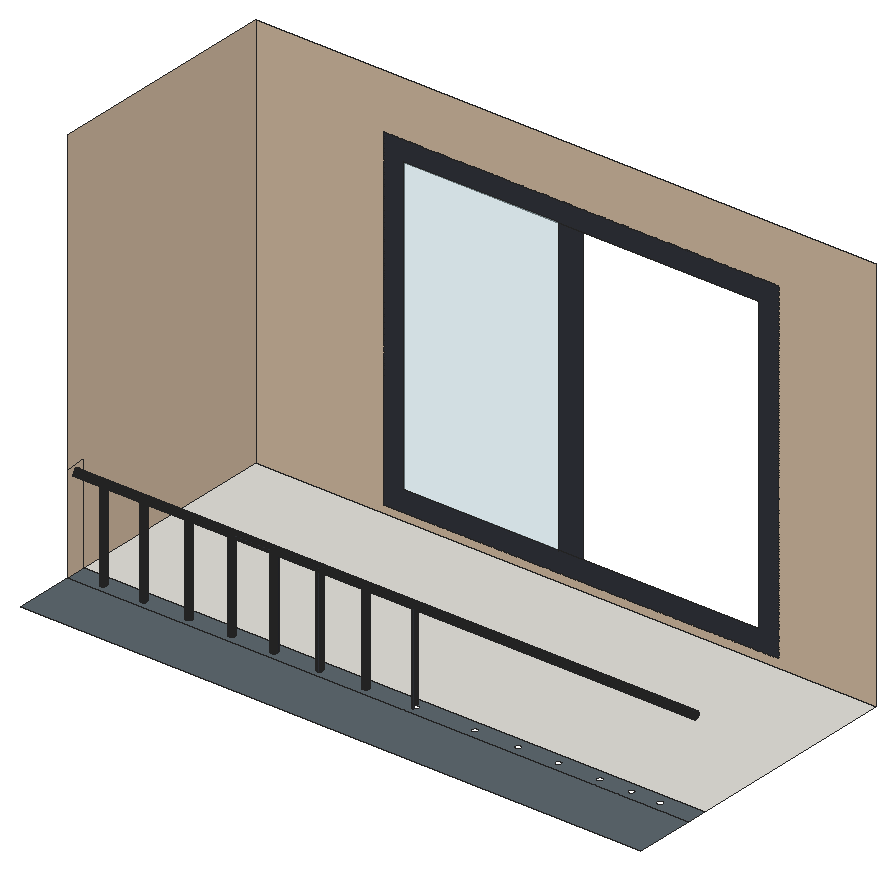
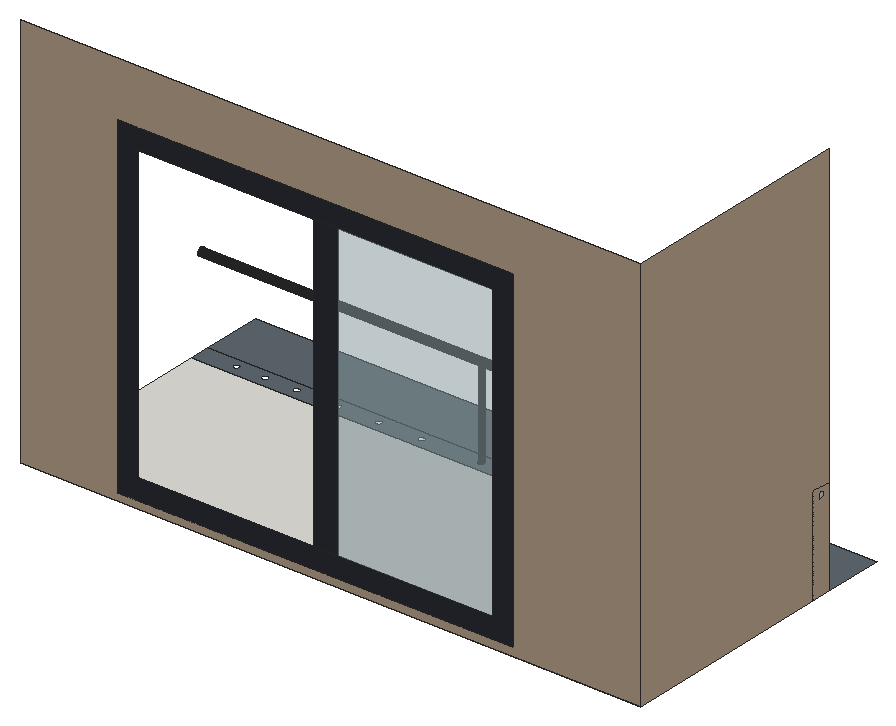
# SketchUp Ruby script. Lengths in inches.
U = 1.inch
M = Sketchup.active_model
def pt(a) = Geom::Point3d.new(a.map { |v| v * U })
def face(e, loops, mat)
  f = e.add_face(loops[0].map { |a| pt(a) })
  loops[1..].each { |l| e.add_face(l.map { |a| pt(a) }).erase! }
  f.material = f.back_material = mat if mat
  f
end
# faces: each face lists its corners as indices into pts; further lists are holes
def faces(e, pts, list, mat = nil) = list.each { |f| face(e, (f[0].is_a?(Array) ? f : [f]).map { |l| l.map { |i| pts[i] } }, mat) }
# xy, xz, yz: faces in a plane at the given z, y or x. An outline is a flat list of corners, or four numbers for a rectangle; further outlines are holes
def ring(l) = l.size == 4 ? [[l[0], l[1]], [l[2], l[1]], [l[2], l[3]], [l[0], l[3]]] : l.each_slice(2).to_a
def flat(e, list, mat, &to3) = list.each { |f| face(e, (f[0].is_a?(Array) ? f : [f]).map { |l| ring(l).map { |u, v| to3.(u, v) } }, mat) }
def xy(e, z, list, mat = nil) = flat(e, list, mat) { |x, y| [x, y, z] }
def xz(e, y, list, mat = nil) = flat(e, list, mat) { |x, z| [x, y, z] }
def yz(e, x, list, mat = nil) = flat(e, list, mat) { |y, z| [x, y, z] }
def lines(e, pts, list) = list.each { |a, b| e.add_line(pt(pts[a]), pt(pts[b])) }
# prism: a flat outline (further loops are holes) pulled along v
def prism(e, loops, v, mat = nil)
  f = face(e, loops, mat); d = Geom::Vector3d.new(v.map { |x| x * U })
  f.pushpull(f.normal.samedirection?(d) ? d.length : -d.length)
end
def box(e, o, s, mat = nil) = prism(e, [[o, [o[0] + s[0], o[1], o[2]], [o[0] + s[0], o[1] + s[1], o[2]], [o[0], o[1] + s[1], o[2]]]], [0, 0, s[2]], mat)
def at(x, y, z, deg = 0) = Geom::Transformation.translation(pt([x, y, z])) * Geom::Transformation.rotation(ORIGIN, Z_AXIS, deg.degrees)
def axes(o, x, y, z) = Geom::Transformation.new([*x, 0, *y, 0, *z, 0, *pt(o).to_a, 1])
def part(name) = M.definitions.add(name)
# library, detail: a bought-in or finely detailed component or shape, given as its bounding box
def library(name, o, s) = part(name).tap { |d| box(d.entities, o, s) }
def detail(e, o, s) = box(e.add_group.entities, o, s)
def put(e, d, t, mat = nil) = e.add_instance(d, t).tap { |i| i.material = mat if mat }
def group(e, t, mat = nil) = e.add_group.tap { |g| g.transformation = t; g.material = mat if mat }.entities
root = M.entities
M.materials.add("[Formica Laminate Dark]").color = [50, 53, 60]
M.materials.add("[Formica Laminate Light]").color = [213, 189, 164]
M.materials.add("[Formica Speckled Grey]").color = [94, 105, 111]
M.materials.add("[Marble Carrara Gold Floor Tile]").color = [225, 223, 217]
M.materials.add("[Translucent Glass Safety]").color = [204, 235, 244]
M.materials["[Translucent Glass Safety]"].alpha = 0.5
xy(root,133.5625,[[17.2,124.59,16.95,124.62,16.73,124.71,16.53,124.86,16.38,125.06,16.29,125.28,16.26,125.52,16.29,125.77,16.38,125.99,16.53,126.1875,16.73,126.34,16.95,126.43,17.2,126.46,17.4375,126.43,17.67,126.34,17.86,126.1875,18.01,125.99,18.1,125.77,18.13,125.52,18.1,125.28,18.01,125.06,17.86,124.86,17.67,124.71,17.4375,124.62],[29.01,124.59,28.77,124.62,28.54,124.71,28.35,124.86,28.2,125.06,28.1,125.28,28.07,125.52,28.1,125.77,28.2,125.99,28.35,126.1875,28.54,126.34,28.77,126.43,29.01,126.46,29.25,126.43,29.48,126.34,29.67,126.1875,29.82,125.99,29.91,125.77,29.95,125.52,29.91,125.28,29.82,125.06,29.67,124.86,29.48,124.71,29.25,124.62],[42.13,124.59,41.89,124.62,41.67,124.71,41.47,124.86,41.32,125.06,41.23,125.28,41.2,125.52,41.23,125.77,41.32,125.99,41.47,126.1875,41.67,126.34,41.89,126.43,42.13,126.46,42.375,126.43,42.6,126.34,42.8,126.1875,42.95,125.99,43.04,125.77,43.07,125.52,43.04,125.28,42.95,125.06,42.8,124.86,42.6,124.71,42.375,124.62],[54.63,124.59,54.39,124.62,54.17,124.71,53.97,124.86,53.82,125.06,53.73,125.28,53.7,125.52,53.73,125.77,53.82,125.99,53.97,126.1875,54.17,126.34,54.39,126.43,54.63,126.46,54.875,126.43,55.1,126.34,55.3,126.1875,55.45,125.99,55.54,125.77,55.57,125.52,55.54,125.28,55.45,125.06,55.3,124.86,55.1,124.71,54.875,124.62],[66.88,124.59,66.64,124.62,66.42,124.71,66.22,124.86,66.07,125.06,65.98,125.28,65.95,125.52,65.98,125.77,66.07,125.99,66.22,126.1875,66.42,126.34,66.64,126.43,66.88,126.46,67.125,126.43,67.35,126.34,67.55,126.1875,67.7,125.99,67.79,125.77,67.82,125.52,67.79,125.28,67.7,125.06,67.55,124.86,67.35,124.71,67.125,124.62],
  [80.2,124.59,79.95,124.62,79.73,124.71,79.53,124.86,79.38,125.06,79.29,125.28,79.26,125.52,79.29,125.77,79.38,125.99,79.53,126.1875,79.73,126.34,79.95,126.43,80.2,126.46,80.4375,126.43,80.67,126.34,80.86,126.1875,81.01,125.99,81.1,125.77,81.13,125.52,81.1,125.28,81.01,125.06,80.86,124.86,80.67,124.71,80.4375,124.62],[93.63,124.59,93.39,124.62,93.17,124.71,92.97,124.86,92.82,125.06,92.73,125.28,92.7,125.52,92.73,125.77,92.82,125.99,92.97,126.1875,93.17,126.34,93.39,126.43,93.63,126.46,93.875,126.43,94.1,126.34,94.3,126.1875,94.45,125.99,94.54,125.77,94.57,125.52,94.54,125.28,94.45,125.06,94.3,124.86,94.1,124.71,93.875,124.62]])
xy(root,133.5625,[[9,105.54,189.57,122.79],[[9,122.79,189.57,128.69],[179.2,124.59,178.95,124.62,178.73,124.71,178.53,124.86,178.38,125.06,178.29,125.28,178.26,125.52,178.29,125.77,178.38,125.99,178.53,126.1875,178.73,126.34,178.95,126.43,179.2,126.46,179.4375,126.43,179.67,126.34,179.86,126.1875,180.01,125.99,180.1,125.77,180.13,125.52,180.1,125.28,180.01,125.06,179.86,124.86,179.67,124.71,179.4375,124.62],[29.01,124.59,28.77,124.62,28.54,124.71,28.35,124.86,28.2,125.06,28.1,125.28,28.07,125.52,28.1,125.77,28.2,125.99,28.35,126.1875,28.54,126.34,28.77,126.43,29.01,126.46,29.25,126.43,29.48,126.34,29.67,126.1875,29.82,125.99,29.91,125.77,29.95,125.52,29.91,125.28,29.82,125.06,29.67,124.86,29.48,124.71,29.25,124.62],[161.7,124.59,161.45,124.62,161.23,124.71,161.03,124.86,160.88,125.06,160.79,125.28,160.76,125.52,160.79,125.77,160.88,125.99,161.03,126.1875,161.23,126.34,161.45,126.43,161.7,126.46,161.9375,126.43,162.17,126.34,162.36,126.1875,162.51,125.99,162.6,125.77,162.63,125.52,162.6,125.28,162.51,125.06,162.36,124.86,162.17,124.71,161.9375,124.62],[42.13,124.59,41.89,124.62,41.67,124.71,41.47,124.86,41.32,125.06,41.23,125.28,41.2,125.52,41.23,125.77,41.32,125.99,41.47,126.1875,41.67,126.34,41.89,126.43,42.13,126.46,42.375,126.43,42.6,126.34,42.8,126.1875,42.95,125.99,43.04,125.77,43.07,125.52,43.04,125.28,42.95,125.06,42.8,124.86,42.6,124.71,42.375,124.62],[149.57,124.59,149.33,124.62,149.1,124.71,148.91,124.86,148.76,125.06,148.67,125.28,148.63,125.52,148.67,125.77,148.76,125.99,148.91,126.1875,149.1,126.34,149.33,126.43,149.57,126.46,149.8125,126.43,150.04,126.34,150.23,126.1875,150.38,125.99,150.48,125.77,150.51,125.52,150.48,125.28,150.38,125.06,150.23,124.86,150.04,124.71,149.8125,124.62],[54.63,124.59,54.39,124.62,54.17,124.71,53.97,124.86,53.82,125.06,53.73,125.28,53.7,125.52,53.73,125.77,53.82,125.99,53.97,126.1875,54.17,126.34,54.39,126.43,54.63,126.46,54.875,126.43,55.1,126.34,55.3,126.1875,55.45,125.99,55.54,125.77,55.57,125.52,55.54,125.28,55.45,125.06,55.3,124.86,55.1,124.71,54.875,124.62],[137.76,124.59,137.52,124.62,137.29,124.71,137.1,124.86,136.95,125.06,136.85,125.28,136.82,125.52,136.85,125.77,136.95,125.99,137.1,126.1875,137.29,126.34,137.52,126.43,137.76,126.46,138,126.43,138.23,126.34,138.42,126.1875,138.57,125.99,138.66,125.77,138.7,125.52,138.66,125.28,138.57,125.06,138.42,124.86,138.23,124.71,138,124.62],[66.88,124.59,66.64,124.62,66.42,124.71,66.22,124.86,66.07,125.06,65.98,125.28,65.95,125.52,65.98,125.77,66.07,125.99,66.22,126.1875,66.42,126.34,66.64,126.43,66.88,126.46,67.125,126.43,67.35,126.34,67.55,126.1875,67.7,125.99,67.79,125.77,67.82,125.52,67.79,125.28,67.7,125.06,67.55,124.86,67.35,124.71,67.125,124.62],[125.32,124.59,125.08,124.62,124.85,124.71,124.66,124.86,124.51,125.06,124.42,125.28,124.38,125.52,124.42,125.77,124.51,125.99,124.66,126.1875,124.85,126.34,125.08,126.43,125.32,126.46,125.5625,126.43,125.79,126.34,125.98,126.1875,126.13,125.99,126.23,125.77,126.26,125.52,126.23,125.28,126.13,125.06,125.98,124.86,125.79,124.71,125.5625,124.62],[80.2,124.59,79.95,124.62,79.73,124.71,79.53,124.86,79.38,125.06,79.29,125.28,79.26,125.52,79.29,125.77,79.38,125.99,79.53,126.1875,79.73,126.34,79.95,126.43,80.2,126.46,80.4375,126.43,80.67,126.34,80.86,126.1875,81.01,125.99,81.1,125.77,81.13,125.52,81.1,125.28,81.01,125.06,80.86,124.86,80.67,124.71,80.4375,124.62],[108.2,124.59,107.95,124.62,107.73,124.71,107.53,124.86,107.38,125.06,107.29,125.28,107.26,125.52,107.29,125.77,107.38,125.99,107.53,126.1875,107.73,126.34,107.95,126.43,108.2,126.46,108.4375,126.43,108.67,126.34,108.86,126.1875,109.01,125.99,109.1,125.77,109.13,125.52,109.1,125.28,109.01,125.06,108.86,124.86,108.67,124.71,108.4375,124.62],[93.63,124.59,93.39,124.62,93.17,124.71,92.97,124.86,92.82,125.06,92.73,125.28,92.7,125.52,92.73,125.77,92.82,125.99,92.97,126.1875,93.17,126.34,93.39,126.43,93.63,126.46,93.875,126.43,94.1,126.34,94.3,126.1875,94.45,125.99,94.54,125.77,94.57,125.52,94.54,125.28,94.45,125.06,94.3,124.86,94.1,124.71,93.875,124.62],[170.82,124.59,170.58,124.62,170.35,124.71,170.16,124.86,170.01,125.06,169.92,125.28,169.88,125.52,169.92,125.77,170.01,125.99,170.16,126.1875,170.35,126.34,170.58,126.43,170.82,126.46,171.0625,126.43,171.29,126.34,171.48,126.1875,171.63,125.99,171.73,125.77,171.76,125.52,171.73,125.28,171.63,125.06,171.48,124.86,171.29,124.71,171.0625,124.62],[17.2,124.59,16.95,124.62,16.73,124.71,16.53,124.86,16.38,125.06,16.29,125.28,16.26,125.52,16.29,125.77,16.38,125.99,16.53,126.1875,16.73,126.34,16.95,126.43,17.2,126.46,17.4375,126.43,17.67,126.34,17.86,126.1875,18.01,125.99,18.1,125.77,18.13,125.52,18.1,125.28,18.01,125.06,17.86,124.86,17.67,124.71,17.4375,124.62]]],"[Formica Speckled Grey]")
xy(root,133.5625,[[9,128.69,189.57,191.15]],"[Marble Carrara Gold Floor Tile]")
xy(root,159.8125,[[29.01,124.59,29.25,124.62,29.48,124.71,29.67,124.86,29.82,125.06,29.91,125.28,29.95,125.52,29.91,125.77,29.82,125.99,29.67,126.1875,29.48,126.34,29.25,126.43,29.01,126.46,28.77,126.43,28.54,126.34,28.35,126.1875,28.2,125.99,28.1,125.77,28.07,125.52,28.1,125.28,28.2,125.06,28.35,124.86,28.54,124.71,28.77,124.62]])
xy(root,159.9375,[[93.63,124.59,93.875,124.62,94.1,124.71,94.3,124.86,94.45,125.06,94.54,125.28,94.57,125.52,94.54,125.77,94.45,125.99,94.3,126.1875,94.1,126.34,93.875,126.43,93.63,126.46,93.39,126.43,93.17,126.34,92.97,126.1875,92.82,125.99,92.73,125.77,92.7,125.52,92.73,125.28,92.82,125.06,92.97,124.86,93.17,124.71,93.39,124.62]])
xy(root,160.19,[[54.63,124.59,54.78,124.61,54.49,124.61],[66.88,124.59,67.03,124.61,66.74,124.61],[54.49,124.61,54.78,124.61,54.875,124.62,55.1,124.71,55.3,124.86,55.45,125.06,55.54,125.28,55.57,125.52,55.54,125.77,55.45,125.99,55.3,126.1875,55.1,126.34,54.875,126.43,54.63,126.46,54.39,126.43,54.17,126.34,53.97,126.1875,53.82,125.99,53.73,125.77,53.7,125.52,53.73,125.28,53.82,125.06,53.97,124.86,54.17,124.71,54.39,124.62],[66.74,124.61,67.03,124.61,67.125,124.62,67.35,124.71,67.55,124.86,67.7,125.06,67.79,125.28,67.82,125.52,67.79,125.77,67.7,125.99,67.55,126.1875,67.35,126.34,67.125,126.43,66.88,126.46,66.64,126.43,66.42,126.34,66.22,126.1875,66.07,125.99,65.98,125.77,65.95,125.52,65.98,125.28,66.07,125.06,66.22,124.86,66.42,124.71,66.64,124.62]])
xy(root,160.25,[[42.13,124.59,42.375,124.62,42.6,124.71,42.8,124.86,42.95,125.06,43.04,125.28,43.07,125.52,43.04,125.77,42.95,125.99,42.8,126.1875,42.6,126.34,42.375,126.43,42.13,126.46,41.89,126.43,41.67,126.34,41.47,126.1875,41.32,125.99,41.23,125.77,41.2,125.52,41.23,125.28,41.32,125.06,41.47,124.86,41.67,124.71,41.89,124.62]])
xy(root,160.4375,[[17.2,124.59,17.4375,124.62,17.67,124.71,17.86,124.86,18.01,125.06,18.1,125.28,18.13,125.52,18.1,125.77,18.01,125.99,17.86,126.1875,17.67,126.34,17.4375,126.43,17.2,126.46,16.95,126.43,16.73,126.34,16.53,126.1875,16.38,125.99,16.29,125.77,16.26,125.52,16.29,125.28,16.38,125.06,16.53,124.86,16.73,124.71,16.95,124.62]])
xy(root,160.625,[[80.2,124.59,80.4375,124.62,80.67,124.71,80.86,124.86,81.01,125.06,81.1,125.28,81.13,125.52,81.1,125.77,81.01,125.99,80.86,126.1875,80.67,126.34,80.4375,126.43,80.2,126.46,79.95,126.43,79.73,126.34,79.53,126.1875,79.38,125.99,79.29,125.77,79.26,125.52,79.29,125.28,79.38,125.06,79.53,124.86,79.73,124.71,79.95,124.62]])
xz(root,191.15,[[[46.38,135.91,161.13,233.1],[52.18,141.71,155.34,227.3]],[97.09,141.71,104.16,227.3]],"[Formica Laminate Dark]")
xz(root,191.15,[[[9,133.5625,189.57,249],[46.38,135.91,161.13,233.1]]],"[Formica Laminate Light]")
xz(root,191.15,[[52.18,141.71,97.09,227.3]],"[Translucent Glass Safety]")
yz(root,9,[[125.67,159.02,125.41,159.03,125.16,159.11,124.94,159.25,124.77,159.45,124.65,159.68,124.59,159.93,124.61,160.19,124.6875,160.44,124.83,160.66,125.02,160.84,125.26,160.96,125.51,161.01,125.77,161,126.02,160.92,126.24,160.77,126.41,160.58,126.53,160.35,126.59,160.09,126.57,159.83,126.49,159.58,126.35,159.36,126.16,159.1875,125.92,159.07]])
yz(root,9,[[128.69,133.5625,191.15,133.5625,191.15,249,122.79,249,122.79,161.92,128.69,162.3125],[[122.79,133.5625,128.69,133.5625,128.69,162.3125,122.79,161.92],[125.67,159.02,125.41,159.03,125.16,159.11,124.94,159.25,124.77,159.45,124.65,159.68,124.59,159.93,124.61,160.19,124.6875,160.44,124.83,160.66,125.02,160.84,125.26,160.96,125.51,161.01,125.77,161,126.02,160.92,126.24,160.77,126.41,160.58,126.53,160.35,126.59,160.09,126.57,159.83,126.49,159.58,126.35,159.36,126.16,159.1875,125.92,159.07]]],"[Formica Laminate Light]")
p = [[16.73,124.71,133.5625],[16.95,124.62,133.5625],[16.95,124.62,160.4375],[16.73,124.71,160.4375],[17.2,124.59,133.5625],[17.2,124.59,160.4375],
  [17.4375,124.62,133.5625],[17.4375,124.62,160.4375],[17.67,124.71,133.5625],[17.67,124.71,160.4375],[28.54,124.71,133.5625],[28.77,124.62,133.5625],
  [28.77,124.62,159.8125],[28.54,124.71,159.8125],[29.01,124.59,133.5625],[29.01,124.59,159.8125],[29.25,124.62,133.5625],[29.25,124.62,159.8125],
  [29.48,124.71,133.5625],[29.48,124.71,159.8125],[41.67,124.71,133.5625],[41.89,124.62,133.5625],[41.89,124.62,160.25],[41.67,124.71,160.25],
  [42.13,124.59,133.5625],[42.13,124.59,160.25],[42.375,124.62,133.5625],[42.375,124.62,160.25],[42.6,124.71,133.5625],[42.6,124.71,160.25],
  [54.17,124.71,133.5625],[54.39,124.62,133.5625],[54.39,124.62,160.19],[54.17,124.71,160.19],[54.63,124.59,133.5625],[54.63,124.59,160.19],
  [54.49,124.61,160.19],[54.875,124.62,133.5625],[54.875,124.62,160.19],[54.78,124.61,160.19],[55.1,124.71,133.5625],[55.1,124.71,160.19],
  [66.42,124.71,133.5625],[66.64,124.62,133.5625],[66.64,124.62,160.19],[66.42,124.71,160.19],[66.88,124.59,133.5625],[66.88,124.59,160.19],
  [66.74,124.61,160.19],[67.125,124.62,133.5625],[67.125,124.62,160.19],[67.03,124.61,160.19],[67.35,124.71,133.5625],[67.35,124.71,160.19],
  [79.73,124.71,133.5625],[79.95,124.62,133.5625],[79.95,124.62,160.625],[79.73,124.71,160.625],[80.2,124.59,133.5625],[80.2,124.59,160.625],
  [80.4375,124.62,133.5625],[80.4375,124.62,160.625],[80.67,124.71,133.5625],[80.67,124.71,160.625],[93.17,124.71,133.5625],[93.39,124.62,133.5625],
  [93.39,124.62,159.9375],[93.17,124.71,159.9375],[93.63,124.59,133.5625],[93.63,124.59,159.9375],[93.875,124.62,133.5625],[93.875,124.62,159.9375],
  [94.1,124.71,133.5625],[94.1,124.71,159.9375],[107.73,124.71,133.5625],[107.95,124.62,133.5625],[107.95,124.62,160.125],[107.73,124.71,160.125],
  [108.2,124.59,133.5625],[108.2,124.59,160.125],[16.53,124.86,133.5625],[16.53,124.86,160.4375],[17.86,124.86,133.5625],[17.86,124.86,160.4375],
  [28.35,124.86,133.5625],[28.35,124.86,159.8125],[29.67,124.86,133.5625],[29.67,124.86,159.8125],[41.47,124.86,133.5625],[41.47,124.86,160.25],
  [42.8,124.86,133.5625],[42.8,124.86,160.25],[53.97,124.86,133.5625],[53.97,124.86,160.19],[55.3,124.86,133.5625],[55.3,124.86,160.19],
  [66.22,124.86,133.5625],[66.22,124.86,160.19],[67.55,124.86,133.5625],[67.55,124.86,160.19],[79.53,124.86,133.5625],[79.53,124.86,160.625],
  [80.86,124.86,133.5625],[80.86,124.86,160.625],[92.97,124.86,133.5625],[92.97,124.86,159.9375],[94.3,124.86,133.5625],[94.3,124.86,159.9375],
  [107.53,124.86,133.5625],[107.53,124.86,160.125],[16.38,125.06,133.5625],[16.38,125.06,160.4375],[18.01,125.06,133.5625],[18.01,125.06,160.4375],
  [28.2,125.06,133.5625],[28.2,125.06,159.8125],[29.82,125.06,133.5625],[29.82,125.06,159.8125],[41.32,125.06,133.5625],[41.32,125.06,160.25],
  [42.95,125.06,133.5625],[42.95,125.06,160.25],[53.82,125.06,133.5625],[53.82,125.06,160.19],[55.45,125.06,133.5625],[55.45,125.06,160.19],
  [66.07,125.06,133.5625],[66.07,125.06,160.19],[67.7,125.06,133.5625],[67.7,125.06,160.19],[79.38,125.06,133.5625],[79.38,125.06,160.625],
  [81.01,125.06,133.5625],[81.01,125.06,160.625],[92.82,125.06,133.5625],[92.82,125.06,159.9375],[94.45,125.06,133.5625],[94.45,125.06,159.9375],
  [107.38,125.06,133.5625],[107.38,125.06,160.125],[16.29,125.28,133.5625],[16.29,125.28,160.4375],[18.1,125.28,133.5625],[18.1,125.28,160.4375],
  [28.1,125.28,133.5625],[28.1,125.28,159.8125],[29.91,125.28,133.5625],[29.91,125.28,159.8125],[41.23,125.28,133.5625],[41.23,125.28,160.25],
  [43.04,125.28,133.5625],[43.04,125.28,160.25],[53.73,125.28,133.5625],[53.73,125.28,160.19],[55.54,125.28,133.5625],[55.54,125.28,160.19],
  [65.98,125.28,133.5625],[65.98,125.28,160.19],[67.79,125.28,133.5625],[67.79,125.28,160.19],[79.29,125.28,133.5625],[79.29,125.28,160.625],
  [81.1,125.28,133.5625],[81.1,125.28,160.625],[92.73,125.28,133.5625],[92.73,125.28,159.9375],[94.54,125.28,133.5625],[94.54,125.28,159.9375],
  [107.29,125.28,133.5625],[107.29,125.28,160.125],[16.26,125.52,133.5625],[16.26,125.52,160.4375],[18.13,125.52,133.5625],[18.13,125.52,160.4375],
  [28.07,125.52,133.5625],[28.07,125.52,159.8125],[29.95,125.52,133.5625],[29.95,125.52,159.8125],[41.2,125.52,133.5625],[41.2,125.52,160.25],
  [43.07,125.52,133.5625],[43.07,125.52,160.25],[53.7,125.52,133.5625],[53.7,125.52,160.19],[55.57,125.52,133.5625],[55.57,125.52,160.19],
  [65.95,125.52,133.5625],[65.95,125.52,160.19],[67.82,125.52,133.5625],[67.82,125.52,160.19],[79.26,125.52,133.5625],[79.26,125.52,160.625],
  [81.13,125.52,133.5625],[81.13,125.52,160.625],[92.7,125.52,133.5625],[92.7,125.52,159.9375],[94.57,125.52,133.5625],[94.57,125.52,159.9375],
  [107.26,125.52,133.5625],[107.26,125.52,160.125],[16.29,125.77,133.5625],[16.29,125.77,160.4375],[18.1,125.77,133.5625],[18.1,125.77,160.4375],
  [28.1,125.77,133.5625],[28.1,125.77,159.8125],[29.91,125.77,133.5625],[29.91,125.77,159.8125],[41.23,125.77,133.5625],[41.23,125.77,160.25],
  [43.04,125.77,133.5625],[43.04,125.77,160.25],[53.73,125.77,133.5625],[53.73,125.77,160.19],[55.54,125.77,133.5625],[55.54,125.77,160.19],
  [65.98,125.77,133.5625],[65.98,125.77,160.19],[67.79,125.77,133.5625],[67.79,125.77,160.19],[79.29,125.77,133.5625],[79.29,125.77,160.625],
  [81.1,125.77,133.5625],[81.1,125.77,160.625],[92.73,125.77,133.5625],[92.73,125.77,159.9375],[94.54,125.77,133.5625],[94.54,125.77,159.9375],
  [107.29,125.77,133.5625],[107.29,125.77,160.125],[16.38,125.99,133.5625],[16.38,125.99,160.4375],[18.01,125.99,133.5625],[18.01,125.99,160.4375],
  [28.2,125.99,133.5625],[28.2,125.99,159.8125],[29.82,125.99,133.5625],[29.82,125.99,159.8125],[41.32,125.99,133.5625],[41.32,125.99,160.25],
  [42.95,125.99,133.5625],[42.95,125.99,160.25],[53.82,125.99,133.5625],[53.82,125.99,160.19],[55.45,125.99,133.5625],[55.45,125.99,160.19],
  [66.07,125.99,133.5625],[66.07,125.99,160.19],[67.7,125.99,133.5625],[67.7,125.99,160.19],[79.38,125.99,133.5625],[79.38,125.99,160.625],
  [81.01,125.99,133.5625],[81.01,125.99,160.625],[92.82,125.99,133.5625],[92.82,125.99,159.9375],[94.45,125.99,133.5625],[94.45,125.99,159.9375],
  [107.38,125.99,133.5625],[107.38,125.99,160.125],[16.53,126.1875,133.5625],[16.53,126.1875,160.4375],[17.86,126.1875,133.5625],[17.86,126.1875,160.4375],
  [28.35,126.1875,133.5625],[28.35,126.1875,159.8125],[29.67,126.1875,133.5625],[29.67,126.1875,159.8125],[41.47,126.1875,133.5625],[41.47,126.1875,160.25],
  [42.8,126.1875,133.5625],[42.8,126.1875,160.25],[53.97,126.1875,133.5625],[53.97,126.1875,160.19],[55.3,126.1875,133.5625],[55.3,126.1875,160.19],
  [66.22,126.1875,133.5625],[66.22,126.1875,160.19],[67.55,126.1875,133.5625],[67.55,126.1875,160.19],[79.53,126.1875,133.5625],[79.53,126.1875,160.625],
  [80.86,126.1875,133.5625],[80.86,126.1875,160.625],[92.97,126.1875,133.5625],[92.97,126.1875,159.9375],[94.3,126.1875,133.5625],[94.3,126.1875,159.9375],
  [107.53,126.1875,133.5625],[107.53,126.1875,160.125],[16.73,126.34,133.5625],[16.73,126.34,160.4375],[17.67,126.34,133.5625],[17.67,126.34,160.4375],
  [28.54,126.34,133.5625],[28.54,126.34,159.8125],[29.48,126.34,133.5625],[29.48,126.34,159.8125],[41.67,126.34,133.5625],[41.67,126.34,160.25],
  [42.6,126.34,133.5625],[42.6,126.34,160.25],[54.17,126.34,133.5625],[54.17,126.34,160.19],[55.1,126.34,133.5625],[55.1,126.34,160.19],
  [66.42,126.34,133.5625],[66.42,126.34,160.19],[67.35,126.34,133.5625],[67.35,126.34,160.19],[79.73,126.34,133.5625],[79.73,126.34,160.625],
  [80.67,126.34,133.5625],[80.67,126.34,160.625],[93.17,126.34,133.5625],[93.17,126.34,159.9375],[94.1,126.34,133.5625],[94.1,126.34,159.9375],
  [107.73,126.34,133.5625],[107.73,126.34,160.125],[16.95,126.43,133.5625],[16.95,126.43,160.4375],[17.4375,126.43,133.5625],[17.4375,126.43,160.4375],
  [28.77,126.43,133.5625],[28.77,126.43,159.8125],[29.25,126.43,133.5625],[29.25,126.43,159.8125],[41.89,126.43,133.5625],[41.89,126.43,160.25],
  [42.375,126.43,133.5625],[42.375,126.43,160.25],[54.39,126.43,133.5625],[54.39,126.43,160.19],[54.875,126.43,133.5625],[54.875,126.43,160.19],
  [66.64,126.43,133.5625],[66.64,126.43,160.19],[67.125,126.43,133.5625],[67.125,126.43,160.19],[79.95,126.43,133.5625],[79.95,126.43,160.625],
  [80.4375,126.43,133.5625],[80.4375,126.43,160.625],[93.39,126.43,133.5625],[93.39,126.43,159.9375],[93.875,126.43,133.5625],[93.875,126.43,159.9375],
  [107.95,126.43,133.5625],[107.95,126.43,160.125],[17.2,126.46,133.5625],[17.2,126.46,160.4375],[29.01,126.46,133.5625],[29.01,126.46,159.8125],
  [42.13,126.46,133.5625],[42.13,126.46,160.25],[54.63,126.46,133.5625],[54.63,126.46,160.19],[66.88,126.46,133.5625],[66.88,126.46,160.19],
  [80.2,126.46,133.5625],[80.2,126.46,160.625],[93.63,126.46,133.5625],[93.63,126.46,159.9375],[9,125.16,159.11],[9,125.41,159.03],
  [189.57,125.41,159.03],[189.57,125.16,159.11],[9,125.67,159.02],[189.57,125.67,159.02],[9,125.92,159.07],[189.57,125.92,159.07],
  [9,124.94,159.25],[189.57,124.94,159.25],[9,126.16,159.1875],[189.57,126.16,159.1875],[9,126.35,159.36],[189.57,126.35,159.36],
  [9,124.77,159.45],[189.57,124.77,159.45],[9,124.65,159.68],[189.57,124.65,159.68],[9,126.49,159.58],[189.57,126.49,159.58],
  [9,126.57,159.83],[189.57,126.57,159.83],[9,124.59,159.93],[189.57,124.59,159.93],[9,126.59,160.09],[189.57,126.59,160.09],
  [9,124.61,160.19],[189.57,124.61,160.19],[170.96,124.61,160.19],[170.68,124.61,160.19],[9,126.53,160.35],[189.57,126.53,160.35],
  [9,124.6875,160.44],[189.57,124.6875,160.44],[9,126.41,160.58],[189.57,126.41,160.58],[9,124.83,160.66],[189.57,124.83,160.66],
  [9,126.24,160.77],[189.57,126.24,160.77],[9,125.02,160.84],[189.57,125.02,160.84],[9,125.26,160.96],[189.57,125.26,160.96],
  [9,126.02,160.92],[189.57,126.02,160.92],[9,125.77,161],[189.57,125.77,161],[9,125.51,161.01],[189.57,125.51,161.01]]
faces(root,p,[[0,1,2,3],[1,4,5,2],[4,6,7,5],[6,8,9,7],[10,11,12,13],[11,14,15,12],[14,16,17,15],[16,18,19,17],
  [20,21,22,23],[21,24,25,22],[24,26,27,25],[26,28,29,27],[30,31,32,33],[31,34,35,36,32],[34,37,38,39,35],[37,40,41,38],
  [42,43,44,45],[43,46,47,48,44],[46,49,50,51,47],[49,52,53,50],[54,55,56,57],[55,58,59,56],[58,60,61,59],[60,62,63,61],
  [64,65,66,67],[65,68,69,66],[68,70,71,69],[70,72,73,71],[74,75,76,77],[75,78,79,76],[80,0,3,81],[8,82,83,9],
  [84,10,13,85],[18,86,87,19],[88,20,23,89],[28,90,91,29],[92,30,33,93],[40,94,95,41],[96,42,45,97],[52,98,99,53],
  [100,54,57,101],[62,102,103,63],[104,64,67,105],[72,106,107,73],[108,74,77,109],[110,80,81,111],[82,112,113,83],[114,84,85,115],
  [86,116,117,87],[118,88,89,119],[90,120,121,91],[122,92,93,123],[94,124,125,95],[126,96,97,127],[98,128,129,99],[130,100,101,131],
  [102,132,133,103],[134,104,105,135],[106,136,137,107],[138,108,109,139],[140,110,111,141],[112,142,143,113],[144,114,115,145],[116,146,147,117],
  [148,118,119,149],[120,150,151,121],[152,122,123,153],[124,154,155,125],[156,126,127,157],[128,158,159,129],[160,130,131,161],[132,162,163,133],
  [164,134,135,165],[136,166,167,137],[168,138,139,169],[170,140,141,171],[142,172,173,143],[174,144,145,175],[146,176,177,147],[178,148,149,179],
  [150,180,181,151],[182,152,153,183],[154,184,185,155],[186,156,157,187],[158,188,189,159],[190,160,161,191],[162,192,193,163],[194,164,165,195],
  [166,196,197,167],[198,168,169,199],[200,170,171,201],[172,202,203,173],[204,174,175,205],[176,206,207,177],[208,178,179,209],[180,210,211,181],
  [212,182,183,213],[184,214,215,185],[216,186,187,217],[188,218,219,189],[220,190,191,221],[192,222,223,193],[224,194,195,225],[196,226,227,197],
  [228,198,199,229],[230,200,201,231],[202,232,233,203],[234,204,205,235],[206,236,237,207],[238,208,209,239],[210,240,241,211],[242,212,213,243],
  [214,244,245,215],[246,216,217,247],[218,248,249,219],[250,220,221,251],[222,252,253,223],[254,224,225,255],[226,256,257,227],[258,228,229,259],
  [260,230,231,261],[232,262,263,233],[264,234,235,265],[236,266,267,237],[268,238,239,269],[240,270,271,241],[272,242,243,273],[244,274,275,245],
  [276,246,247,277],[248,278,279,249],[280,250,251,281],[252,282,283,253],[284,254,255,285],[256,286,287,257],[288,258,259,289],[290,260,261,291],
  [262,292,293,263],[294,264,265,295],[266,296,297,267],[298,268,269,299],[270,300,301,271],[302,272,273,303],[274,304,305,275],[306,276,277,307],
  [278,308,309,279],[310,280,281,311],[282,312,313,283],[314,284,285,315],[286,316,317,287],[318,288,289,319],[320,290,291,321],[292,322,323,293],
  [324,294,295,325],[296,326,327,297],[328,298,299,329],[300,330,331,301],[332,302,303,333],[304,334,335,305],[336,306,307,337],[308,338,339,309],
  [340,310,311,341],[312,342,343,313],[344,314,315,345],[316,346,347,317],[348,318,319,349],[350,320,321,351],[322,350,351,323],[352,324,325,353],
  [326,352,353,327],[354,328,329,355],[330,354,355,331],[356,332,333,357],[334,356,357,335],[358,336,337,359],[338,358,359,339],[360,340,341,361],
  [342,360,361,343],[362,344,345,363],[346,362,363,347],[364,365,366,367],[365,368,369,366],[368,370,371,369],[372,364,367,373],[370,374,375,371],
  [374,376,377,375],[378,372,373,379],[380,378,379,381],[376,382,383,377],[382,384,385,383],[386,380,381,387],[384,388,389,385],[390,386,387,391,392,393,51,48,39,36],
  [388,394,395,389],[396,390,36,39,48,51,393,392,391,397],[394,398,399,395],[400,396,397,401],[398,402,403,399],[404,400,401,405],[406,404,405,407],[402,408,409,403],
  [408,410,411,409],[412,406,407,413],[410,412,413,411]],"[Formica Laminate Dark]")
